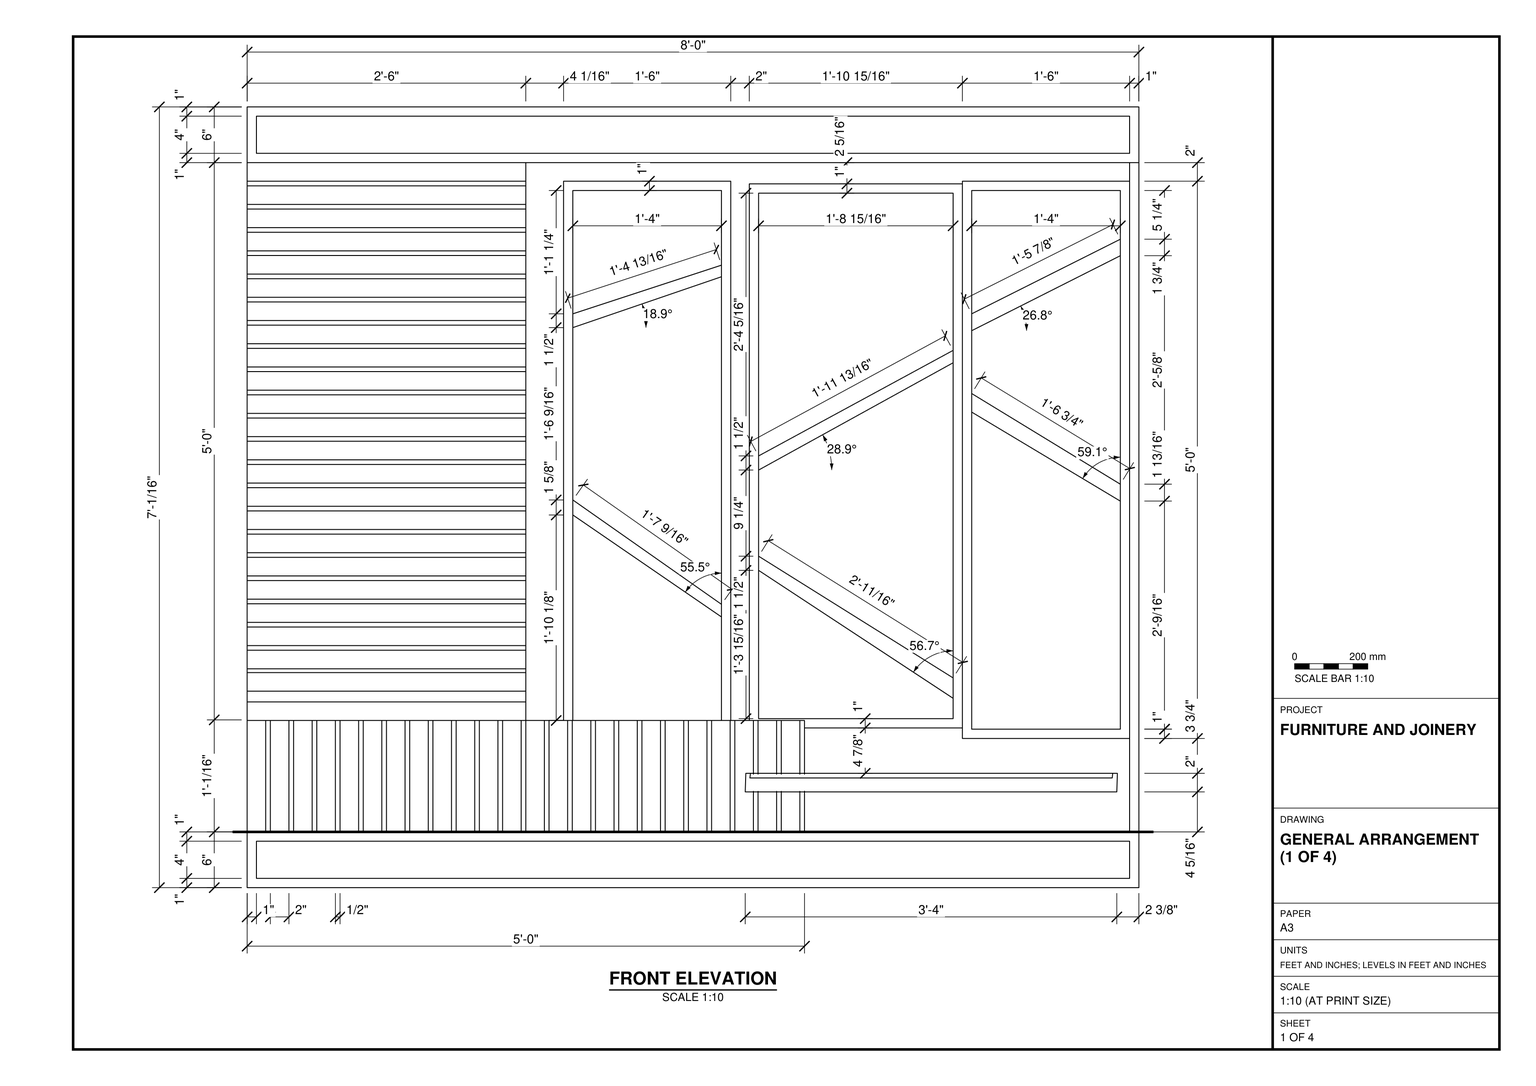
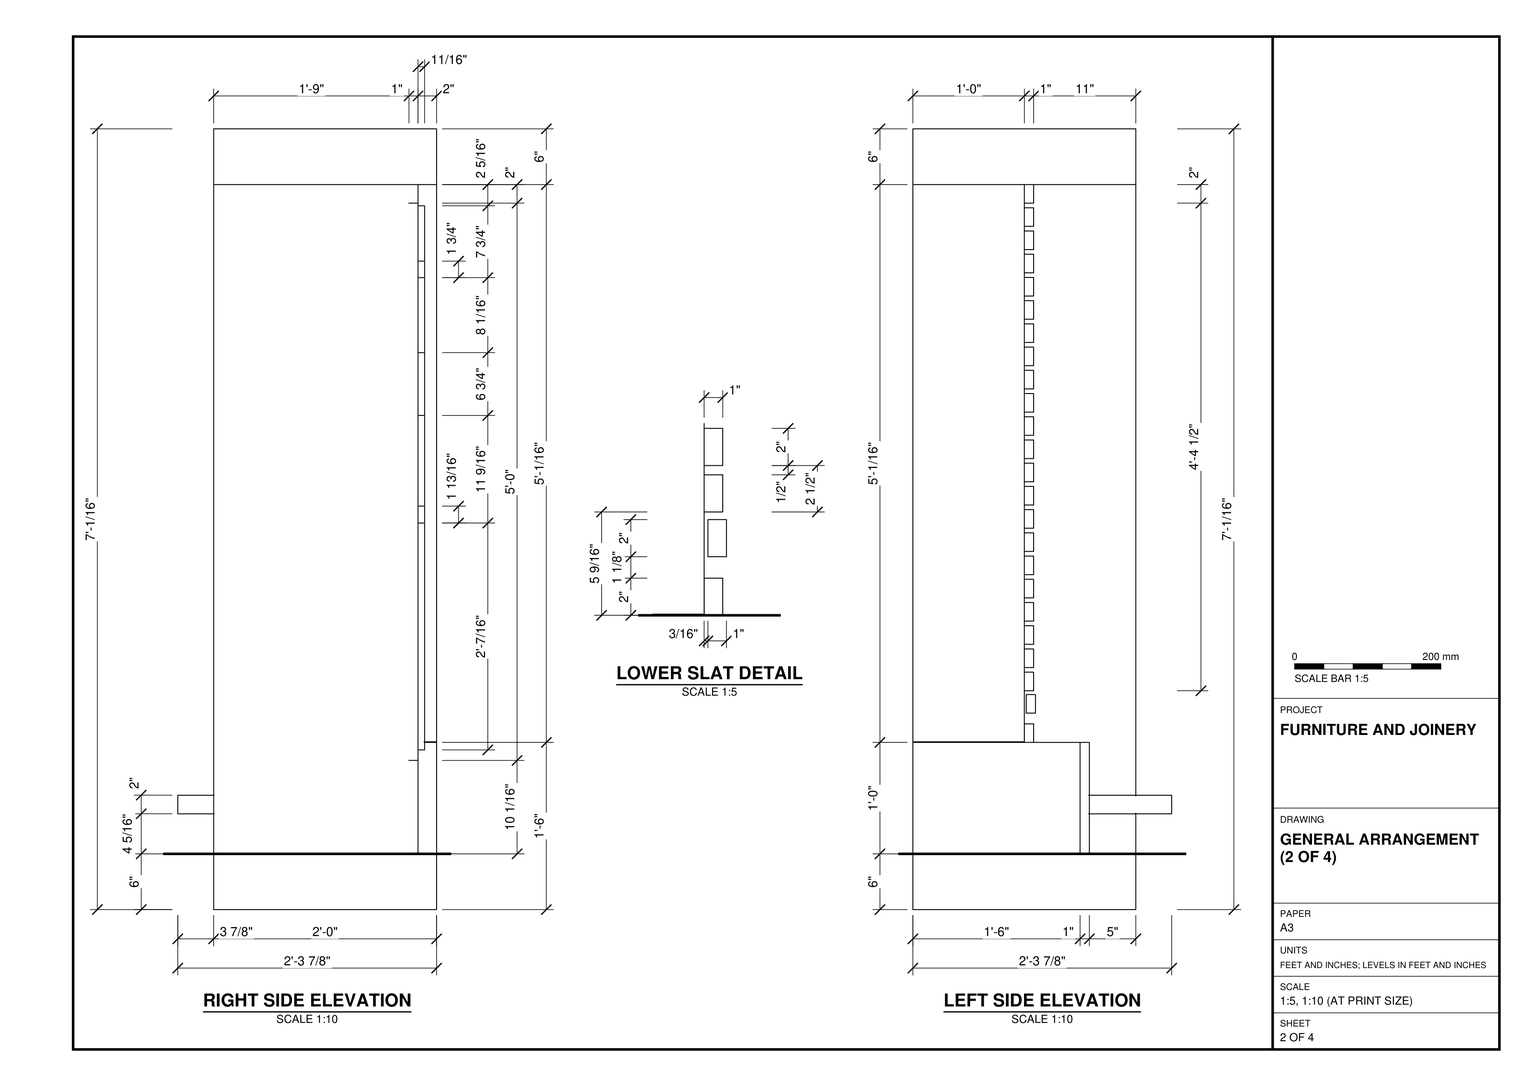
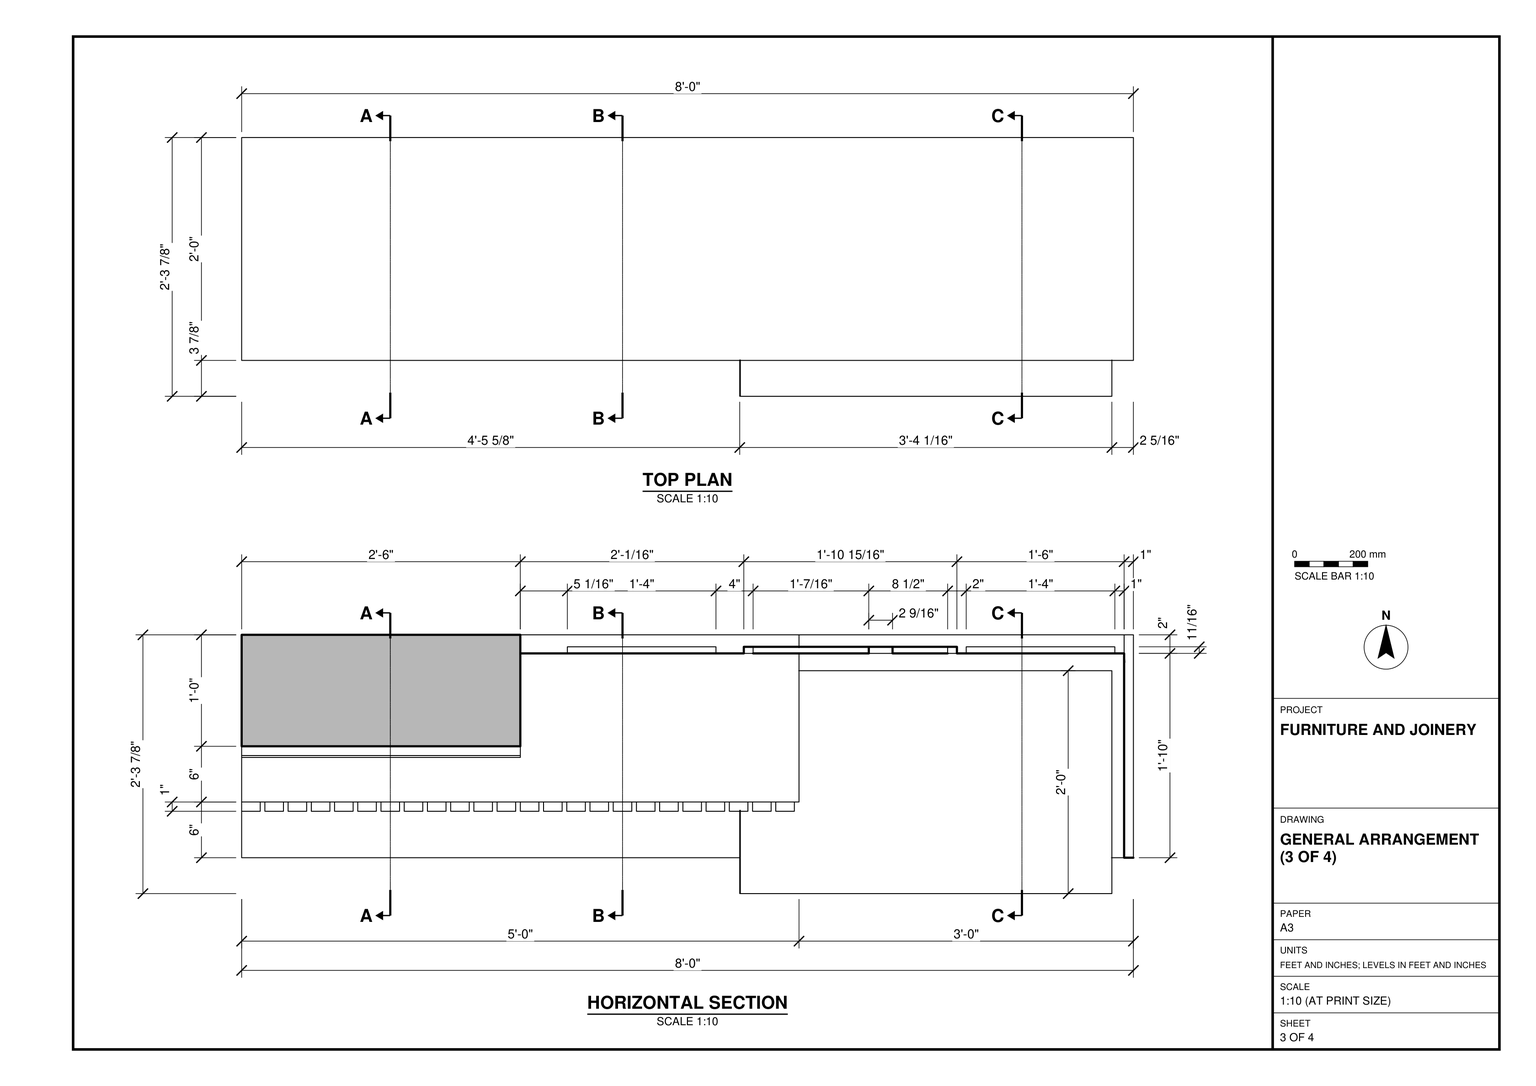
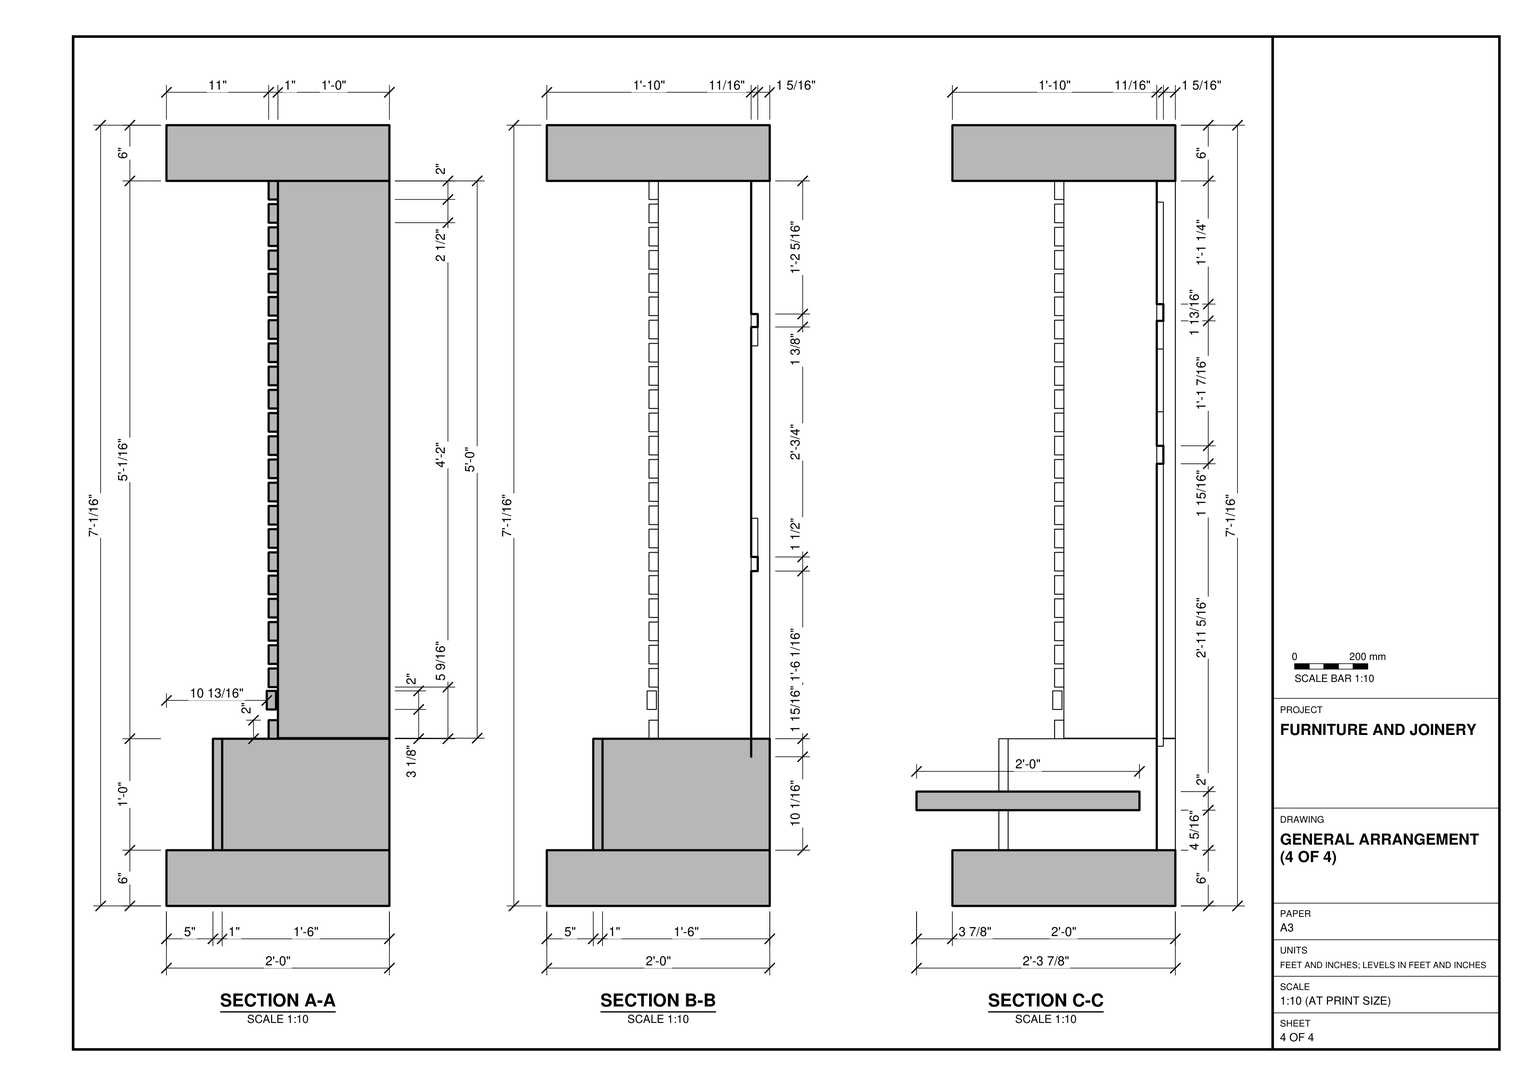
Build the display unit in SketchUp from task_files/diagram_01.pdf. Work in feet and inches, with the underside of the base at ±0'-0". The finished unit is 8'-0" wide, 2'-3 7/8" deep including the projecting ledge, and 7'-1/16" high.

Model the full-width top and base bands with the narrow borders shown in the front elevation. On the left, build a tall field of horizontal slats above a lower field of vertical slats. The lower field extends farther to the right and sits forward of the upper field. Use the horizontal section and side elevations to set these depth changes; model the slats with thickness and gaps rather than drawing lines on a face.

To the right of the upper slats, form three tall framed bays. Make the middle bay wider than its neighbours and follow the elevation for the slope and endpoint of each diagonal shelf. Include the right end return and the low ledge that projects beyond the base. Group distinct joinery pieces separately and use components for repeated parts. Any decor or loose items shown may use suitable library components. Save one SketchUp model as output_files/slatted_display_unit_with_diagonal_shelves.skp.

# SketchUp Ruby script. Lengths in inches.
U = 1.inch
M = Sketchup.active_model
def pt(a) = Geom::Point3d.new(a.map { |v| v * U })
def face(e, loops, mat)
  f = e.add_face(loops[0].map { |a| pt(a) })
  loops[1..].each { |l| e.add_face(l.map { |a| pt(a) }).erase! }
  f.material = f.back_material = mat if mat
  f
end
# faces: each face lists its corners as indices into pts; further lists are holes
def faces(e, pts, list, mat = nil) = list.each { |f| face(e, (f[0].is_a?(Array) ? f : [f]).map { |l| l.map { |i| pts[i] } }, mat) }
# xy, xz, yz: faces in a plane at the given z, y or x. An outline is a flat list of corners, or four numbers for a rectangle; further outlines are holes
def ring(l) = l.size == 4 ? [[l[0], l[1]], [l[2], l[1]], [l[2], l[3]], [l[0], l[3]]] : l.each_slice(2).to_a
def flat(e, list, mat, &to3) = list.each { |f| face(e, (f[0].is_a?(Array) ? f : [f]).map { |l| ring(l).map { |u, v| to3.(u, v) } }, mat) }
def xy(e, z, list, mat = nil) = flat(e, list, mat) { |x, y| [x, y, z] }
def xz(e, y, list, mat = nil) = flat(e, list, mat) { |x, z| [x, y, z] }
def yz(e, x, list, mat = nil) = flat(e, list, mat) { |y, z| [x, y, z] }
def lines(e, pts, list) = list.each { |a, b| e.add_line(pt(pts[a]), pt(pts[b])) }
# prism: a flat outline (further loops are holes) pulled along v
def prism(e, loops, v, mat = nil)
  f = face(e, loops, mat); d = Geom::Vector3d.new(v.map { |x| x * U })
  f.pushpull(f.normal.samedirection?(d) ? d.length : -d.length)
end
def box(e, o, s, mat = nil) = prism(e, [[o, [o[0] + s[0], o[1], o[2]], [o[0] + s[0], o[1] + s[1], o[2]], [o[0], o[1] + s[1], o[2]]]], [0, 0, s[2]], mat)
def at(x, y, z, deg = 0) = Geom::Transformation.translation(pt([x, y, z])) * Geom::Transformation.rotation(ORIGIN, Z_AXIS, deg.degrees)
def axes(o, x, y, z) = Geom::Transformation.new([*x, 0, *y, 0, *z, 0, *pt(o).to_a, 1])
def part(name) = M.definitions.add(name)
# library, detail: a bought-in or finely detailed component or shape, given as its bounding box
def library(name, o, s) = part(name).tap { |d| box(d.entities, o, s) }
def detail(e, o, s) = box(e.add_group.entities, o, s)
def put(e, d, t, mat = nil) = e.add_instance(d, t).tap { |i| i.material = mat if mat }
def group(e, t, mat = nil) = e.add_group.tap { |g| g.transformation = t; g.material = mat if mat }.entities
root = M.entities
box(root,[0,14.86,76.0625],[30,1,2])
box(root,[0,14.86,73.5625],[30,1,2])
box(root,[0,14.86,71.0625],[30,1,2])
box(root,[0,14.86,68.5625],[30,1,2])
box(root,[0,14.86,66.0625],[30,1,2])
box(root,[0,14.86,63.5625],[30,1,2])
box(root,[0,14.86,61.0625],[30,1,2])
box(root,[0,14.86,58.5625],[30,1,2])
box(root,[0,14.86,56.0625],[30,1,2])
box(root,[0,14.86,53.5625],[30,1,2])
box(root,[0,14.86,51.0625],[30,1,2])
box(root,[0,14.86,48.5625],[30,1,2])
box(root,[0,14.86,46.0625],[30,1,2])
box(root,[0,14.86,43.5625],[30,1,2])
box(root,[0,14.86,41.0625],[30,1,2])
box(root,[0,14.86,38.5625],[30,1,2])
box(root,[0,14.86,36.0625],[30,1,2])
box(root,[0,14.86,33.5625],[30,1,2])
box(root,[0,14.86,31.0625],[30,1,2])
box(root,[0,14.86,28.5625],[30,1,2])
box(root,[0,14.86,26.0625],[30,1,2])
box(root,[0,14.86,23.5625],[30,1,2])
box(root,[0,14.66,21.15],[30,1,2])
g1 = group(root,at(0,27.86,18.0625))
box(g1,[0,-12,0],[30,12,60])
g2 = group(root,at(0,3.86,0))
g3 = group(g2,at(0,0,0))
xy(g3,0,[[0,0,96,24]])
xy(g3,6,[[0,0,95,0,95,22,60,22,60,6,59.5,6,59.5,5,57.5,5,57.5,6,57,6,57,5,55,5,55,6,54.5,6,54.5,5,52.5,5,52.5,6,52,6,52,5,50,5,50,6,49.5,6,49.5,5,47.5,5,47.5,6,47,6,47,5,45,5,45,6,44.5,6,44.5,5,42.5,5,42.5,6,42,6,42,5,40,5,40,6,39.5,6,39.5,5,37.5,5,37.5,6,37,6,37,5,35,5,35,6,34.5,6,34.5,5,32.5,5,32.5,6,32,6,32,5,30,5,30,6,29.5,6,29.5,5,27.5,5,27.5,6,27,6,27,5,25,5,25,6,24.5,6,24.5,5,22.5,5,22.5,6,22,6,22,5,20,5,20,6,19.5,6,19.5,5,17.5,5,17.5,6,17,6,17,5,15,5,15,6,14.5,6,14.5,5,12.5,5,12.5,6,12,6,12,5,10,5,10,6,9.5,6,9.5,5,7.5,5,7.5,6,7,6,7,5,5,5,5,6,4.5,6,4.5,5,2.5,5,2.5,6,2,6,2,5,0,5],[95,0,96,24],[0,5,2,6],[2.5,5,4.5,6],[5,5,7,6],
  [7.5,5,9.5,6],[10,5,12,6],[12.5,5,14.5,6],[15,5,17,6],[17.5,5,19.5,6],
  [20,5,22,6],[22.5,5,24.5,6],[25,5,27,6],[27.5,5,29.5,6],[30,5,32,6],
  [32.5,5,34.5,6],[35,5,37,6],[37.5,5,39.5,6],[40,5,42,6],[42.5,5,44.5,6],
  [45,5,47,6],[47.5,5,49.5,6],[50,5,52,6],[52.5,5,54.5,6],[55,5,57,6],
  [57.5,5,59.5,6],[0,6,60,24],[60,22,95,24]])
xy(g3,10.3125,[[53.62,-3.86,93.62,20.14]])
xy(g3,12.3125,[[53.68,-3.86,93.68,20.14]])
xy(g3,17.2,[[60,22,77,22.71]])
xy(g3,18,[[0,5,2,6],[2.5,5,4.5,6],[5,5,7,6],[7.5,5,9.5,6],[10,5,12,6],
  [12.5,5,14.5,6],[15,5,17,6],[17.5,5,19.5,6],[20,5,22,6],[22.5,5,24.5,6],
  [25,5,27,6],[27.5,5,29.5,6],[30,5,32,6],[32.5,5,34.5,6],[35,5,37,6],
  [37.5,5,39.5,6],[40,5,42,6],[42.5,5,44.5,6],[45,5,47,6],[47.5,5,49.5,6],
  [50,5,52,6],[52.5,5,54.5,6],[55,5,57,6],[57.5,5,59.5,6],[0,6,60,6,60,22,30,22,30,24,0,24,0,12,30,12,30,11,0,11],
  [0,11,30,12],[30,22,54.06,22,54.06,22.71,60,22.71,60,24,30,24],[54.06,22,60,22.71]])
xy(g3,20,[[0,11,30,12]])
xy(g3,75.78,[[54.06,22,77,22.71]])
xy(g3,78.0625,[[0,0,0,24,30,24,30,22,95,22,95,0],[95,0,96,24],[30,22,95,24]])
xy(g3,84.0625,[[0,0,96,24]])
xz(g3,-3.86,[[53.62,10.3125,93.62,10.3125,93.68,12.3125,93.18,12.3125,93.12,11.8125,54.12,11.8125,54.18,12.3125,53.68,12.3125],[54.12,11.8125,93.12,11.8125,93.18,12.3125,54.18,12.3125]])
xz(g3,0,[[[0,0,96,6],[1,1,95,5]],[1,1,95,5],[95,6,96,78.0625],[[0,78.0625,96,84.0625],[1,79.0625,95,83.0625]],[1,79.0625,95,83.0625]])
xz(g3,5,[[0,6,2,18],[2.5,6,4.5,18],[5,6,7,18],[7.5,6,9.5,18],[10,6,12,18],
  [12.5,6,14.5,18],[15,6,17,18],[17.5,6,19.5,18],[20,6,22,18],[22.5,6,24.5,18],
  [25,6,27,18],[27.5,6,29.5,18],[30,6,32,18],[32.5,6,34.5,18],[35,6,37,18],
  [37.5,6,39.5,18],[40,6,42,18],[42.5,6,44.5,18],[45,6,47,18],[47.5,6,49.5,18],
  [50,6,52,18],[52.5,6,54.5,18],[55,6,57,18],[57.5,6,59.5,18]])
xz(g3,6,[[0,6,2,18],[2,6,2.5,18],[2.5,6,4.5,18],[4.5,6,5,18],[5,6,7,18],
  [7,6,7.5,18],[7.5,6,9.5,18],[9.5,6,10,18],[10,6,12,18],[12,6,12.5,18],
  [12.5,6,14.5,18],[14.5,6,15,18],[15,6,17,18],[17,6,17.5,18],[17.5,6,19.5,18],
  [19.5,6,20,18],[20,6,22,18],[22,6,22.5,18],[22.5,6,24.5,18],[24.5,6,25,18],
  [25,6,27,18],[27,6,27.5,18],[27.5,6,29.5,18],[29.5,6,30,18],[30,6,32,18],
  [32,6,32.5,18],[32.5,6,34.5,18],[34.5,6,35,18],[35,6,37,18],[37,6,37.5,18],
  [37.5,6,39.5,18],[39.5,6,40,18],[40,6,42,18],[42,6,42.5,18],[42.5,6,44.5,18],
  [44.5,6,45,18],[45,6,47,18],[47,6,47.5,18],[47.5,6,49.5,18],[49.5,6,50,18],
  [50,6,52,18],[52,6,52.5,18],[52.5,6,54.5,18],[54.5,6,55,18],[55,6,57,18],
  [57,6,57.5,18],[57.5,6,59.5,18],[59.5,6,60,18]])
xz(g3,11,[[0,18,30,20]])
xz(g3,12,[[0,18,30,20]])
xz(g3,20.14,[[53.62,10.3125,53.68,12.3125,93.68,12.3125,93.62,10.3125]])
xz(g3,22,[[60,6,60,17.2,77,17.2,77,16.0625,95,16.0625,95,6],[[34.0625,16.0625,52.0625,76.0625],[35.0625,17.0625,51.0625,75.0625]],[[77,16.0625,95,76.0625],[78,17.0625,94,75.0625]],[35.0625,17.0625,51.0625,18],[78,17.0625,78,51.2,94,41.62,94,17.0625],
  [54.06,17.2,60,18],[30,18,30,78.0625,95,78.0625,95,76.0625,77,76.0625,77,75.78,54.06,75.78,54.06,18,52.0625,18,52.0625,76.0625,34.0625,76.0625,34.0625,18],[34.0625,18,34.0625,76.0625,52.0625,76.0625,52.0625,18,51.0625,18,51.0625,75.0625,35.0625,75.0625,35.0625,18],[35.0625,18,35.0625,40.13,51.0625,29.15,51.0625,18],[55.06,18.2,55.06,34.16,76,20.39,76,18.2],
  [76,22.58,55.06,35.6875,55.06,44.96,76,56.52],[51.0625,30.51,35.0625,41.74,35.0625,60.3,51.0625,65.78],[94,43.44,78,53.2,78,59.97,94,68.04],[55.06,46.49,55.06,74.78,76,74.78,76,57.85],[35.0625,61.78,35.0625,75.0625,51.0625,75.0625,51.0625,67.03],
  [78,61.78,78,75.0625,94,75.0625,94,69.82]])
xz(g3,22.71,[[[60,17.2,60,18,54.06,18,54.06,75.78,77,75.78,77,17.2],[76,20.39,76,22.58,55.06,35.6875,55.06,34.16],[55.06,44.96,76,56.52,76,57.85,55.06,46.49]],[51.0625,29.15,35.0625,40.13,35.0625,41.74,51.0625,30.51],[94,41.62,78,51.2,78,53.2,94,43.44],[55.06,44.96,55.06,46.49,76,57.85,76,56.52],[78,59.97,78,61.78,94,69.82,94,68.04],
  [35.0625,60.3,35.0625,61.78,51.0625,67.03,51.0625,65.78]])
xz(g3,24,[[0,0,96,6],[0,6,30,18],[30,6,60,18],[0,18,30,18.0625],[0,78.0625,96,84.0625]])
yz(g3,0,[[0,0,24,6],[5,6,6,18],[6,6,24,18],[11,18,12,20],[0,78.0625,24,84.0625]])
yz(g3,2,[[5,6,6,18]])
yz(g3,2.5,[[5,6,6,18]])
yz(g3,4.5,[[5,6,6,18]])
yz(g3,5,[[5,6,6,18]])
yz(g3,7,[[5,6,6,18]])
yz(g3,7.5,[[5,6,6,18]])
yz(g3,9.5,[[5,6,6,18]])
yz(g3,10,[[5,6,6,18]])
yz(g3,12,[[5,6,6,18]])
yz(g3,12.5,[[5,6,6,18]])
yz(g3,14.5,[[5,6,6,18]])
yz(g3,15,[[5,6,6,18]])
yz(g3,17,[[5,6,6,18]])
yz(g3,17.5,[[5,6,6,18]])
yz(g3,19.5,[[5,6,6,18]])
yz(g3,20,[[5,6,6,18]])
yz(g3,22,[[5,6,6,18]])
yz(g3,22.5,[[5,6,6,18]])
yz(g3,24.5,[[5,6,6,18]])
yz(g3,25,[[5,6,6,18]])
yz(g3,27,[[5,6,6,18]])
yz(g3,27.5,[[5,6,6,18]])
yz(g3,29.5,[[5,6,6,18]])
yz(g3,30,[[5,6,6,18],[11,18,12,20],[22,18,24,18.0625],[22,18.0625,24,78.0625]])
yz(g3,32,[[5,6,6,18]])
yz(g3,32.5,[[5,6,6,18]])
yz(g3,34.5,[[5,6,6,18]])
yz(g3,35,[[5,6,6,18]])
yz(g3,35.0625,[[22,40.13,22.71,41.74],[22,60.3,22.71,61.78]])
yz(g3,37,[[5,6,6,18]])
yz(g3,37.5,[[5,6,6,18]])
yz(g3,39.5,[[5,6,6,18]])
yz(g3,40,[[5,6,6,18]])
yz(g3,42,[[5,6,6,18]])
yz(g3,42.5,[[5,6,6,18]])
yz(g3,44.5,[[5,6,6,18]])
yz(g3,45,[[5,6,6,18]])
yz(g3,47,[[5,6,6,18]])
yz(g3,47.5,[[5,6,6,18]])
yz(g3,49.5,[[5,6,6,18]])
yz(g3,50,[[5,6,6,18]])
yz(g3,51.0625,[[22,29.15,22.71,30.51],[22,65.78,22.71,67.03]])
yz(g3,52,[[5,6,6,18]])
yz(g3,52.5,[[5,6,6,18]])
yz(g3,54.06,[[22,18,22.71,75.78]])
yz(g3,54.5,[[5,6,6,18]])
yz(g3,55,[[5,6,6,18]])
yz(g3,55.06,[[22,34.16,22.71,35.6875],[22,44.96,22.71,46.49]])
yz(g3,57,[[5,6,6,18]])
yz(g3,57.5,[[5,6,6,18]])
yz(g3,59.5,[[5,6,6,18]])
yz(g3,60,[[6,6,22,18],[22,6,24,6,24,18,22.71,18,22.71,17.2,22,17.2],[22,17.2,22.71,18]])
yz(g3,76,[[22,20.39,22.71,22.58],[22,56.52,22.71,57.85]])
yz(g3,77,[[22,17.2,22.71,75.78]])
yz(g3,78,[[22,51.2,22.71,53.2],[22,59.97,22.71,61.78]])
yz(g3,94,[[22,41.62,22.71,43.44],[22,68.04,22.71,69.82]])
yz(g3,95,[[0,6,22,78.0625]])
yz(g3,96,[[0,0,24,6],[0,78.0625,24,84.0625]])
p = [[53.62,20.14,10.3125],[53.62,-3.86,10.3125],[53.68,-3.86,12.3125],[53.68,20.14,12.3125],[93.62,-3.86,10.3125],[93.62,20.14,10.3125],
  [93.68,20.14,12.3125],[93.68,-3.86,12.3125],[76,22,20.39],[55.06,22,34.16],[55.06,22.71,34.16],[76,22.71,20.39],
  [55.06,22,35.6875],[76,22,22.58],[76,22.71,22.58],[55.06,22.71,35.6875],[51.0625,22,29.15],[35.0625,22,40.13],
  [35.0625,22.71,40.13],[51.0625,22.71,29.15],[35.0625,22,41.74],[51.0625,22,30.51],[51.0625,22.71,30.51],[35.0625,22.71,41.74],
  [94,22,41.62],[78,22,51.2],[78,22.71,51.2],[94,22.71,41.62],[78,22,53.2],[94,22,43.44],
  [94,22.71,43.44],[78,22.71,53.2],[76,22,56.52],[55.06,22,44.96],[55.06,22.71,44.96],[76,22.71,56.52],
  [55.06,22,46.49],[76,22,57.85],[76,22.71,57.85],[55.06,22.71,46.49],[94,22,68.04],[78,22,59.97],
  [78,22.71,59.97],[94,22.71,68.04],[51.0625,22,65.78],[35.0625,22,60.3],[35.0625,22.71,60.3],[51.0625,22.71,65.78],
  [35.0625,22,61.78],[51.0625,22,67.03],[51.0625,22.71,67.03],[35.0625,22.71,61.78],[78,22,61.78],[94,22,69.82],
  [94,22.71,69.82],[78,22.71,61.78],[95,22,16.0625],[95.09,21,16.0625],[95,22,76.0625],[95.09,21,76.0625]]
faces(g3,p,[[0,1,2,3],[4,5,6,7],[8,9,10,11],[12,13,14,15],[16,17,18,19],[20,21,22,23],[24,25,26,27],[28,29,30,31],
  [32,33,34,35],[36,37,38,39],[40,41,42,43],[44,45,46,47],[48,49,50,51],[52,53,54,55]])
lines(g3,p,[[56,57],[58,59]])
